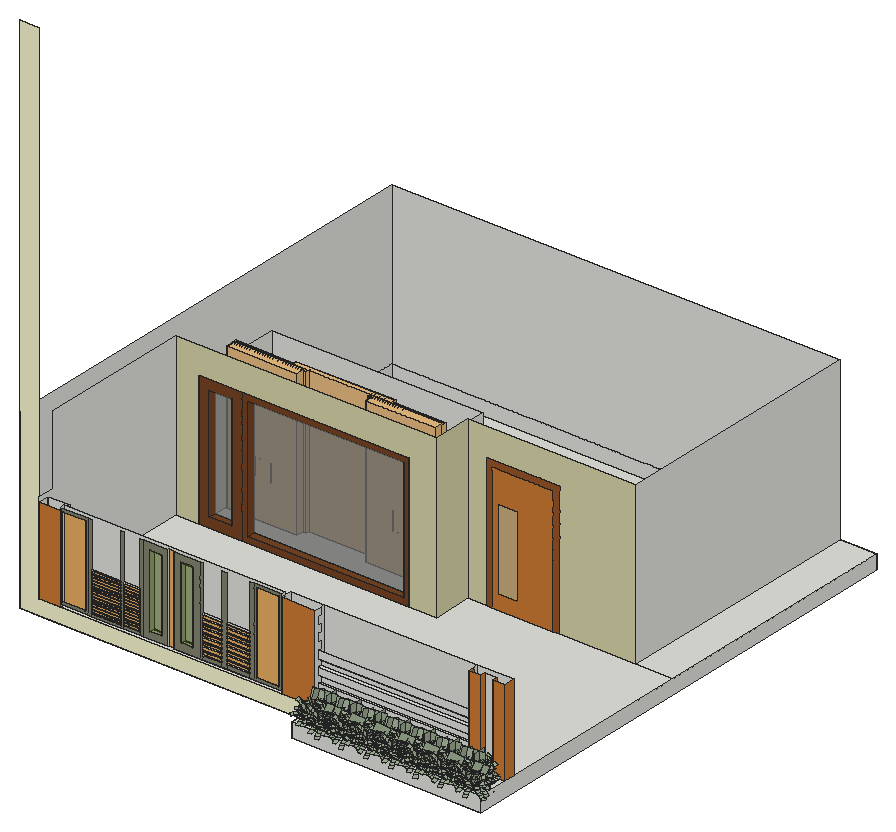
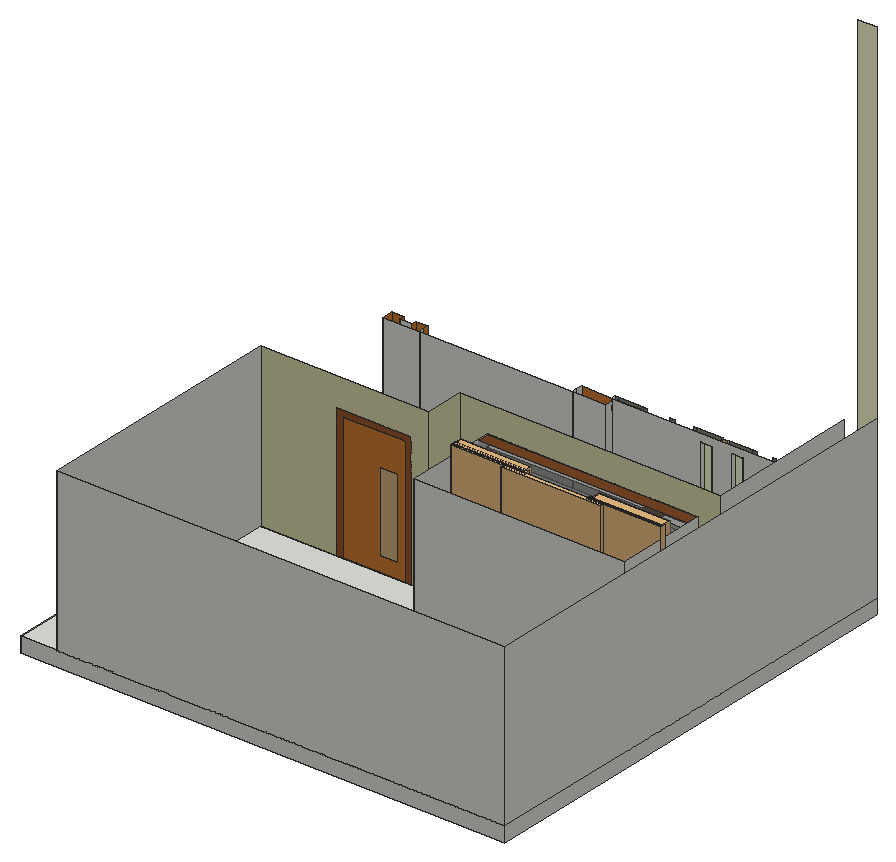
# SketchUp Ruby script. Lengths in inches.
U = 1.inch
M = Sketchup.active_model
def pt(a) = Geom::Point3d.new(a.map { |v| v * U })
def face(e, loops, mat)
  f = e.add_face(loops[0].map { |a| pt(a) })
  loops[1..].each { |l| e.add_face(l.map { |a| pt(a) }).erase! }
  f.material = f.back_material = mat if mat
  f
end
# faces: each face lists its corners as indices into pts; further lists are holes
def faces(e, pts, list, mat = nil) = list.each { |f| face(e, (f[0].is_a?(Array) ? f : [f]).map { |l| l.map { |i| pts[i] } }, mat) }
# xy, xz, yz: faces in a plane at the given z, y or x. An outline is a flat list of corners, or four numbers for a rectangle; further outlines are holes
def ring(l) = l.size == 4 ? [[l[0], l[1]], [l[2], l[1]], [l[2], l[3]], [l[0], l[3]]] : l.each_slice(2).to_a
def flat(e, list, mat, &to3) = list.each { |f| face(e, (f[0].is_a?(Array) ? f : [f]).map { |l| ring(l).map { |u, v| to3.(u, v) } }, mat) }
def xy(e, z, list, mat = nil) = flat(e, list, mat) { |x, y| [x, y, z] }
def xz(e, y, list, mat = nil) = flat(e, list, mat) { |x, z| [x, y, z] }
def yz(e, x, list, mat = nil) = flat(e, list, mat) { |y, z| [x, y, z] }
def lines(e, pts, list) = list.each { |a, b| e.add_line(pt(pts[a]), pt(pts[b])) }
# prism: a flat outline (further loops are holes) pulled along v
def prism(e, loops, v, mat = nil)
  f = face(e, loops, mat); d = Geom::Vector3d.new(v.map { |x| x * U })
  f.pushpull(f.normal.samedirection?(d) ? d.length : -d.length)
end
def box(e, o, s, mat = nil) = prism(e, [[o, [o[0] + s[0], o[1], o[2]], [o[0] + s[0], o[1] + s[1], o[2]], [o[0], o[1] + s[1], o[2]]]], [0, 0, s[2]], mat)
def at(x, y, z, deg = 0) = Geom::Transformation.translation(pt([x, y, z])) * Geom::Transformation.rotation(ORIGIN, Z_AXIS, deg.degrees)
def axes(o, x, y, z) = Geom::Transformation.new([*x, 0, *y, 0, *z, 0, *pt(o).to_a, 1])
def part(name) = M.definitions.add(name)
# library, detail: a bought-in or finely detailed component or shape, given as its bounding box
def library(name, o, s) = part(name).tap { |d| box(d.entities, o, s) }
def detail(e, o, s) = box(e.add_group.entities, o, s)
def put(e, d, t, mat = nil) = e.add_instance(d, t).tap { |i| i.material = mat if mat }
def group(e, t, mat = nil) = e.add_group.tap { |g| g.transformation = t; g.material = mat if mat }.entities
root = M.entities
M.materials.add("Generic").color = [133, 133, 113]
M.materials.add("Generic\#1").color = [235, 176, 99]
M.materials.add("Generic\#4").color = [217, 213, 170]
M.materials.add("Generic\#7").color = [249, 247, 208]
M.materials.add("[Translucent Glass Dark Green]").color = [62, 91, 5]
M.materials["[Translucent Glass Dark Green]"].alpha = 0.5
M.materials.add("[Translucent Glass Gray]").color = [128, 128, 128]
M.materials["[Translucent Glass Gray]"].alpha = 0.5
M.materials.add("[Wood Bamboo]").color = [206, 124, 53]
M.materials.add("[Wood Cherry Original]").color = [152, 86, 42]
M.materials.add("[Wood Floor Light]").color = [204, 176, 127]
M.materials.add("[Wood Veneer 01]").color = [119, 69, 36]
M.materials.add("hymenocallis littoralis").color = [156, 172, 146]
c1 = part("Group\#856")
xy(c1.entities,7.38,[[0,0,5.5,15.91]],"hymenocallis littoralis")
p = [[5.5,28.78,0],[5.5,26.79,3.44],[0,26.79,3.44],[0,28.78,0],[0,23.75,6],[5.5,23.75,6],
  [0,15.91,7.38],[5.5,15.91,7.38]]
faces(c1.entities,p,[[0,1,2,3],[4,2,1,5],[6,4,5,7]],"hymenocallis littoralis")
c2 = part("Group\#854")
xy(c2.entities,7.38,[[0,0,5.5,15.91],[0,15.91,5.5,23.87]],"hymenocallis littoralis")
p = [[5.5,31.07,4.3],[5.5,27.74,6.47],[0,27.74,6.47],[0,31.07,4.3],[0,23.87,7.38],[5.5,23.87,7.38]]
faces(c2.entities,p,[[0,1,2,3],[4,2,1,5]],"hymenocallis littoralis")
c3 = part("Group\#857")
xy(c3.entities,7.38,[[0,0,5.6,15.91]],"hymenocallis littoralis")
p = [[5.6,28.78,0],[5.6,26.79,3.44],[0,26.79,3.44],[0,28.78,0],[0,23.75,6],[5.6,23.75,6],
  [0,15.91,7.38],[5.6,15.91,7.38]]
faces(c3.entities,p,[[0,1,2,3],[4,2,1,5],[6,4,5,7]],"hymenocallis littoralis")
c4 = part("Group\#855")
put(c4.entities,c2,axes([6.09,8.57,-0.52],[0.446,0.85617,0.26089],[-0.18444,-0.19731,0.96283],[0.87582,-0.47754,0.0699]))
put(c4.entities,c2,axes([6.29,7.28,-1.71],[0.37058,0.92707,-0.05667],[-0.32382,0.19004,0.99128],[0.87712,-0.32925,0.34964]))
put(c4.entities,c2,axes([11.04,16.14,-0.7],[1,0,0],[0,0.16628,1.02662],[0,-1.18456,0.19186]))
c5 = part("Group\#860")
put(c5.entities,c1,axes([24.57,32.05,-1.76],[0.9552,-0.22102,-0.19681],[0.4036,0.95545,0.88585],[-0.00568,-0.67859,0.7345]))
put(c5.entities,c1,axes([23.95,29.24,-2.4],[0,1,0],[-0.76041,0,0.64945],[0.64945,0,0.76041]))
put(c5.entities,c1,axes([24.22,24.72,-0.48],[-0.70711,0.70711,0],[-0.32757,-0.32757,0.80237],[0.61237,0.61237,0.5]))
put(c5.entities,c2,axes([20.66,37.22,-0.63],[1.12361,0.03262,0.39091],[-0.43499,0.29739,0.78777],[0.09852,-1.27434,0.37535]))
put(c5.entities,c1,axes([28.75,24.45,-2.4],[-1,0,0],[0,-0.76041,0.64945],[0,0.64945,0.76041]))
put(c5.entities,c3,axes([30.4,30.98,-3.7],[0.65676,-0.72002,0.22414],[0.55667,0.66341,0.5],[-0.50871,-0.20361,0.83652]))
put(c5.entities,c3,axes([32.41,29.61,-3.7],[0.04029,-0.97372,0.22414],[0.85287,0.15038,0.5],[-0.52057,0.17102,0.83652]))
put(c5.entities,c1,axes([31.89,25.85,-1.76],[-0.92056,0.33739,-0.19681],[-0.5186,-0.89824,0.88585],[0.08952,0.67268,0.7345]))
put(c5.entities,c1,axes([25.55,34.78,-0.48],[0.86603,0.5,0],[-0.25,0.43301,0.86603],[0.43301,-0.75,0.5]))
put(c5.entities,c3,axes([20.4,16.9375,-8.07],[-0.70711,0.70711,0],[-0.35754,-0.35754,0.65422],[1.3987,1.3987,1.52882]))
put(c5.entities,c1,axes([32.86,34.14,-0.48],[0.76604,-0.64279,0],[0.32139,0.38302,0.86603],[-0.55667,-0.66341,0.5]))
put(c5.entities,c1,axes([27.15,34.7,-0.1],[0.82472,-0.17528,-0.53769],[0.53769,0.53769,0.64945],[0.17528,-0.82472,0.53769]))
put(c5.entities,c1,axes([33.58,28.77,-2.4],[0,-1,0],[0.76041,0,0.64945],[-0.64945,0,0.76041]))
put(c5.entities,c1,axes([26.43,23.87,-2.81],[-0.75126,0.04415,0.65853],[0.53769,-0.53769,0.64945],[0.38276,0.84199,0.3802]))
put(c5.entities,c1,axes([28.78,23.98,-2.4],[-1,0,0],[0,-0.76041,0.64945],[0,0.64945,0.76041]))
put(c5.entities,c1,axes([25.39,25.38,-2.4],[-0.70711,0.70711,0],[-0.53769,-0.53769,0.64945],[0.45923,0.45923,0.76041]))
put(c5.entities,c1,axes([27.32,21.63,-0.1],[-0.45923,0.70711,-0.53769],[-0.76041,0,0.64945],[0.45923,0.70711,0.53769]))
put(c5.entities,c1,axes([25.17,27.625,-1.76],[0.56416,0.80187,-0.19681],[-0.66673,0.66673,0.80532],[0.62659,-0.26057,0.7345]))
put(c5.entities,c3,axes([27.59,27.04,-3.96],[-0.8993,-0.06127,0.43301],[0.2962,-0.8138,0.5],[0.32175,0.57791,0.75]))
put(c5.entities,c3,axes([26.98,24.5,-3.18],[-0.5,0.86603,0],[-0.75,-0.43301,0.5],[0.43301,0.25,0.86603]))
put(c5.entities,c3,axes([24.55,27.74,-3.7],[0.29517,0.92878,0.22414],[-0.85287,0.15038,0.5],[0.43068,-0.33875,0.83652]))
put(c5.entities,c3,axes([24.26,29.8,-3.18],[0.76604,0.64279,0],[-0.47317,0.5639,0.425],[0.32139,-0.38302,0.86603]))
put(c5.entities,c3,axes([25.98,32.46,-3.18],[1,0,0],[0,0.86603,0.5],[0,-0.5,0.86603]))
put(c5.entities,c1,axes([28.78,33.57,-2.4],[1,0,0],[0,0.76041,0.64945],[0,-0.64945,0.76041]))
put(c5.entities,c4,at(14.99,21.38,2.5))
put(c5.entities,c2,axes([34.63,26.34,-1.46],[-0.70089,-0.70877,0.07994],[0.4756,-0.38088,0.79293],[-0.53156,0.59378,0.60405]))
put(c5.entities,c2,axes([28.14,16.92,1.8125],[-1.19719,0.6912,0],[-0.09607,-0.16641,0.94244],[0.68444,1.18549,0.17613]))
put(c5.entities,c2,axes([31.5625,35.84,0.97],[0.66765,-1.1564,0.35779],[0.04445,0.30732,0.91033],[-1.20828,-0.64496,0.17012]))
put(c5.entities,c2,axes([38.94,22.51,0.89],[-0.97932,-0.67164,-0.05202],[0.27787,-0.41401,0.90999],[-0.85985,0.93577,0.32097]))
put(c5.entities,c2,axes([38.44,21.09,1.98],[-1.02864,-0.54856,0.2395],[0.33481,0.06999,0.88388],[-0.77261,1.08328,0.06417]))
put(c5.entities,c3,axes([35.02,30.51,-1.3],[-0.17365,-0.98481,0],[0.60224,-0.10619,0.79122],[-0.7792,0.13739,0.61153]))
put(c5.entities,c3,axes([29.41,22.33,-1.3],[-0.93969,0.34202,0],[-0.20915,-0.57465,0.79122],[0.27061,0.74351,0.61153]))
put(c5.entities,c2,axes([19.64,36,-1.62],[1.18194,0.09546,0.08234],[-0.14377,0.68823,0.76313],[0.21457,-1.1326,0.62386]))
put(c5.entities,c3,axes([24.25,24.14,-1.3],[-0.34202,0.93969,0],[-0.57465,-0.20915,0.79122],[0.74351,0.27061,0.61153]))
put(c5.entities,c3,axes([25.98,34.61,-1.3],[1,0,0],[0,0.61153,0.79122],[0,-0.79122,0.61153]))
put(c5.entities,c3,axes([31.16,34.41,-1.64],[0.56518,-0.80224,-0.19234],[0.73413,0.34233,0.72935],[-0.47639,-0.50772,0.71782]))
put(c5.entities,c3,axes([40.52,26.84,-5.82],[-0.42262,-0.90631,0],[0.48019,-0.22391,0.68552],[-1.43418,0.66877,1.22305]))
put(c5.entities,c1,axes([29.86,38.42,-1.01],[0.89064,-0.37013,0.26413],[-0.03924,0.63286,1.01918],[-0.45353,-0.76487,0.45748]))
put(c5.entities,c1,axes([29.34,22.4,-0.48],[-0.99619,-0.08716,0],[0.04358,-0.4981,0.86603],[-0.07548,0.86273,0.5]))
c6 = part("Group\#858")
xz(c6.entities,10.07,[[9.07,0,10.07,31.01],[0,31.01,0,45.12,20.13,45.12,20.13,31.01,10.07,31.01,10.07,32.58,9.07,32.58,9.07,31.01]],"hymenocallis littoralis")
yz(c6.entities,10.07,[[0,31.01,20.13,45.12]],"hymenocallis littoralis")
p = [[9.57,9.2,0],[10.07,10.07,0],[10.07,10.07,31.01],[10.07,10.07,32.58],[9.57,9.2,32.58]]
faces(c6.entities,p,[[0,1,2,3,4]],"hymenocallis littoralis")
c7 = part("cây lá nắng")
put(c7.entities,c5,axes([49.26,-2.75,0],[0.63109,0.63109,0],[-0.63109,0.63109,0],[0,0,0.935]))
g1 = group(c7.entities,at(26.6,-8.68,0))
put(g1,c1,axes([-4.72,35.73,-1.65],[0.74231,0.46334,-0.18402],[-0.34827,0.85768,0.82827],[0.42467,-0.43184,0.68675]))
put(g1,c1,axes([-3.34,33.57,-2.24],[-0.63109,0.63109,0],[-0.47989,-0.47989,0.60723],[0.40986,0.40986,0.71098]))
put(g1,c1,axes([-0.3125,30.89,-0.45],[-0.8925,0,0],[0,-0.41345,0.75022],[0,0.77293,0.4675]))
put(g1,c2,axes([-10.79,39.66,-0.59],[0.68852,0.72969,0.3655],[-0.4622,-0.08684,0.73657],[0.86641,-0.74205,0.35095]))
put(g1,c1,axes([2.71,33.57,-2.24],[-0.63109,-0.63109,0],[0.47989,-0.47989,0.60723],[-0.40986,0.40986,0.71098]))
put(g1,c3,axes([-0.37,38.74,-3.46],[0.86887,-0.03992,0.20957],[-0.06737,0.76999,0.4675],[-0.19255,-0.44954,0.78214]))
put(g1,c3,axes([1.76,39.14,-3.46],[0.63993,-0.58908,0.20957],[0.44333,0.63315,0.4675],[-0.43646,-0.2206,0.78214]))
put(g1,c1,axes([3.81,36.4375,-1.65],[-0.79389,-0.36803,-0.18402],[0.23959,-0.89415,0.82827],[-0.36803,0.48102,0.68675]))
put(g1,c1,axes([-5.83,38.07,-0.45],[0.231,0.86209,0],[-0.43104,0.1155,0.80973],[0.74659,-0.20005,0.4675]))
put(g1,c3,axes([2.18,23.5625,-7.55],[-0.8925,0,0],[0,-0.45128,0.6117],[0,1.76542,1.42944]))
put(g1,c1,axes([-0.8125,42.28,-0.45],[0.8891,0.07779,0],[-0.03889,0.44455,0.80973],[0.06737,-0.76999,0.4675]))
put(g1,c1,axes([-4.76,39.03,-0.09],[0.63109,0.40986,-0.50274],[0,0.67866,0.60723],[0.63109,-0.40986,0.50274]))
put(g1,c1,axes([3.03,39.35,-2.24],[0.63109,-0.63109,0],[0.47989,0.47989,0.60723],[-0.40986,-0.40986,0.71098]))
put(g1,c1,axes([1.61,31.74,-2.625],[-0.50198,-0.44625,0.61573],[0.67866,0,0.60723],[-0.28982,0.77293,0.35549]))
put(g1,c1,axes([3.03,33.3,-2.24],[-0.63109,-0.63109,0],[0.47989,-0.47989,0.60723],[-0.40986,0.40986,0.71098]))
put(g1,c1,axes([0.01,32.04,-2.24],[-0.8925,0,0],[0,-0.67866,0.60723],[0,0.57963,0.71098]))
put(g1,c1,axes([3.59,30.89,-0.09],[-0.73607,0.15643,-0.50274],[-0.47989,-0.47989,0.60723],[-0.15643,0.73607,0.50274]))
put(g1,c1,axes([-1.55,33.32,-1.65],[-0.15002,0.86209,-0.18402],[-0.84154,0,0.75297],[0.55988,0.231,0.68675]))
put(g1,c3,axes([0.35,34.48,-3.71],[-0.52887,-0.60621,0.40487],[0.70051,-0.32665,0.4675],[-0.16166,0.56777,0.70125]))
put(g1,c3,axes([2.61,39.13,-1.74],[-0.86209,0.231,0],[-0.23031,-0.85954,0.15531],[0.03162,0.11799,0.91645]))
put(g1,c3,axes([-2.02,33,-3.46],[-0.39986,0.77243,0.20957],[-0.63315,-0.44333,0.4675],[0.48558,0.05802,0.78214]))
put(g1,c3,axes([-3.49,34.12,-2.97],[0.07779,0.8891,0],[-0.65449,0.05726,0.39737],[0.44455,-0.03889,0.80973]))
put(g1,c3,axes([-4.09,36.88,-2.97],[0.63109,0.63109,0],[-0.54654,0.54654,0.4675],[0.31555,-0.31555,0.80973]))
put(g1,c1,axes([-3.02,39.35,-2.24],[0.63109,0.63109,0],[-0.47989,0.47989,0.60723],[0.40986,-0.40986,0.71098]))
put(g1,c4,axes([-4.03,22.95,2.33],[0.63109,0.63109,0],[-0.63109,0.63109,0],[0,0,0.935]))
put(g1,c2,axes([5.24,38.48,-1.37],[0.00497,-0.88963,0.07474],[0.54052,0.05978,0.74139],[-0.71019,0.03927,0.56479]))
put(g1,c2,axes([7.08,28.4375,1.7],[-1.19175,-0.31933,0],[0.04439,-0.16565,0.88118],[-0.31621,1.1801,0.16468]))
put(g1,c2,axes([-2.7,42.54,0.91],[1.15114,-0.30845,0.33454],[-0.1659,0.22199,0.85115],[-0.3555,-1.16957,0.15907]))
put(g1,c2,axes([10.37,38.78,0.83],[-0.19417,-1.04191,-0.04864],[0.43664,-0.08592,0.85084],[-1.1332,0.04791,0.30011]))
put(g1,c2,axes([10.95,37.5625,1.85],[-0.30298,-0.99536,0.22393],[0.16713,0.25547,0.82643],[-1.17124,0.19607,0.06]))
put(g1,c3,axes([2.84,41.36,-1.22],[0.51192,-0.73109,0],[0.44708,0.31305,0.73979],[-0.57846,-0.40504,0.57178]))
put(g1,c3,axes([4.47,32.65,-1.22],[-0.80888,-0.37719,0],[0.23066,-0.49465,0.73979],[-0.29844,0.64,0.57178]))
put(g1,c2,axes([-10.32,35.12,-1.51],[0.68567,0.80616,0.07699],[-0.52507,0.3436,0.71352],[0.85019,-0.57936,0.58331]))
put(g1,c3,axes([0.07,30.54,-1.22],[-0.80888,0.37719,0],[-0.23066,-0.49465,0.73979],[0.29844,0.64,0.57178]))
put(g1,c3,axes([-5.45,38.24,-1.22],[0.63109,0.63109,0],[-0.38593,0.38593,0.73979],[0.49934,-0.49934,0.57178]))
put(g1,c3,axes([-2.05,41.38,-1.53],[0.86296,-0.14961,-0.17984],[0.24726,0.67935,0.68194],[0.01977,-0.62107,0.67116]))
put(g1,c3,axes([8.63,42.51,-5.4375],[0.30525,-0.83868,0],[0.44435,0.16173,0.64096],[-1.32716,-0.48305,1.14356]))
put(g1,c1,axes([-5.4,43.09,-0.94],[0.79566,0.32849,0.24696],[-0.42416,0.37462,0.95293],[0.19648,-0.76892,0.42774]))
put(g1,c1,axes([4.38,32.65,-0.45],[-0.57369,-0.68369,0],[0.34185,-0.28684,0.80973],[-0.5921,0.49683,0.4675]))
put(g1,c3,axes([-2,33.84,-0.15],[-0.24601,0.85793,0],[-0.85539,-0.24528,0.15531],[0.11742,0.03367,0.91645]))
put(g1,c3,axes([0.17,30.83,-4.47],[-0.24601,0.85793,0],[-0.85539,-0.24528,0.15531],[0.11742,0.03367,0.91645]))
put(g1,c3,axes([-1.97,32.18,-4.47],[0.58524,0.67383,0],[-0.67184,0.58351,0.15531],[0.09222,-0.0801,0.91645]))
put(g1,c3,axes([-2,34.71,-4.47],[0.88392,-0.12346,0],[0.12309,0.88131,0.15531],[-0.0169,-0.12098,0.91645]))
put(g1,c3,axes([0.11,36.12,-4.47],[0.37822,-0.8084,0],[0.80601,0.37711,0.15531],[-0.11064,-0.05177,0.91645]))
put(c7.entities,c6,axes([29.71,14.29,6.94],[0.425,0.73612,0],[-0.6771,0.39092,-0.33349],[-0.26859,0.15507,0.72712]))
put(c7.entities,c6,axes([42.0625,26.12,6.94],[0.85,0,0],[0,0.78185,-0.33349],[0,0.33349,0.78185]))
put(c7.entities,c5,axes([7.3125,23.0625,0],[0.8925,0,0],[0,0.8925,0],[0,0,0.935]))
put(c7.entities,c6,axes([24.4375,40.23,2.05],[0.85,0,0],[0,0.85,0],[0,0,0.85]))
c8 = part("Planting+101")
put(c8.entities,c7,axes([21.34,32.96,-4.59],[0,-0.71,0],[-0.71,0,0],[0,0,0.71]))
c9 = library("Group14",[-64.97,9.24,0.31],[138.52,9.93,292.57])
c10 = library("Group16",[86.37,-10.76,76.46],[21.79,14.87,35.97])
c11 = library("Group22",[48.82,-10.91,0.23],[97.72,18.57,293.12])
c12 = library("Group24",[44.03,2.01,0.26],[103.73,11,292.35])
c13 = library("Group27",[-106.21,-10.76,76.46],[21.8,14.87,35.97])
c14 = library("Group35",[-145.81,2.01,0.26],[103.73,11,292.35])
c15 = library("Group33",[-144.59,-10.91,0.23],[97.72,18.57,293.12])
c16 = part("rem (1)")
g2 = group(c16.entities,at(-145.81,-10.91,0.23))
put(g2,c9,at(145.81,10.91,-0.23))
put(g2,c10,at(145.81,10.91,-0.23))
put(g2,c11,at(145.81,10.91,-0.23))
put(g2,c12,at(145.81,10.91,-0.23))
put(g2,c13,at(145.81,10.91,-0.23))
put(g2,c14,at(145.81,10.91,-0.23))
put(g2,c15,at(145.81,10.91,-0.23))
c17 = part("Group\#5")
xz(c17.entities,0,[[0,0,11.45,75.29]],"[Translucent Glass Dark Green]")
xy(root,-37.25,[[304.6875,37.125,304.6875,67.875,19.1875,67.875,19.1875,244.125,500.125,244.125,500.125,37.125],[0,67.875,0,547.875,500.125,547.875,500.125,244.125,19.1875,244.125,19.1875,67.875]])
xy(root,-29.125,[[309.97,40.97,494.84,64.03]])
xy(root,-21.875,[[[304.6875,37.125,500.125,37.125,500.125,67.875,487.6875,67.875,487.6875,73.0625,475.25,73.0625,475.25,67.875,462.8125,67.875,462.8125,71.375,304.6875,71.375],[309.97,40.97,494.84,64.03]],[19.1875,67.875,41.625,79.3125],[41.625,67.875,269.875,79.3125],[269.875,67.875,304.6875,79.3125],[462.8125,67.875,475.25,67.875,475.25,73.0625,487.6875,73.0625,487.6875,67.875,500.125,67.875,500.125,79.3125,462.8125,79.3125],
  [304.6875,71.375,462.8125,73.0625],[304.6875,73.0625,462.8125,79.3125],[19.1875,79.3125,500.125,79.3125,500.125,284.5625,288.89,284.5625,288.89,244.125,19.1875,244.125],[43.125,244.125,260.5625,338.6875],[462.8125,284.5625,500.125,547.875]])
xy(root,-18.875,[[41.625,67.875,41.625,72.625,269.875,72.625,269.875,67.875,158.75,67.875,158.75,68.625,152.75,68.625,152.75,67.875]])
xy(root,-16.375,[[304.6875,71.375,462.8125,74.375]])
xy(root,-16.14,[[44.36,67.875,67.42,68.625]])
xy(root,-16.125,[[74.16,67.875,103.6875,68.625],[107.25,67.875,123.28,68.625]])
xy(root,-16.11,[[244.11,67.875,267.11,68.625]])
xy(root,-15.3125,[[188.84,67.875,208,68.625],[212.8125,67.875,236.91,68.625]],"Generic")
xy(root,-14.875,[[74.16,67.875,103.6875,68.625],[107.25,67.875,123.28,68.625]])
xy(root,-13.5,[[188.84,67.875,208,68.625],[212.8125,67.875,236.91,68.625]],"Generic")
xy(root,-13.125,[[74.16,67.875,103.6875,68.625],[107.25,67.875,123.28,68.625]])
xy(root,-11.875,[[74.16,67.875,103.6875,68.625],[107.25,67.875,123.28,68.625]])
xy(root,-11.83,[[134.26,67.875,145.71,72.625]])
xy(root,-11.3125,[[166.3125,67.875,177.72,72.625]])
xy(root,-11.125,[[188.84,67.875,208,68.625],[212.8125,67.875,236.91,68.625]],"Generic")
xy(root,-10.125,[[74.16,67.875,103.6875,68.625],[107.25,67.875,123.28,68.625]])
xy(root,-9.3125,[[188.84,67.875,208,68.625],[212.8125,67.875,236.91,68.625]],"Generic")
xy(root,-8.9375,[[304.6875,71.375,462.8125,74.375]])
xy(root,-8.875,[[74.16,67.875,103.6875,68.625],[107.25,67.875,123.28,68.625]])
xy(root,-7.125,[[74.16,67.875,103.6875,68.625],[107.25,67.875,123.28,68.625]])
xy(root,-6.9375,[[188.84,67.875,208,68.625],[212.8125,67.875,236.91,68.625]],"Generic")
xy(root,-5.875,[[74.16,67.875,103.6875,68.625],[107.25,67.875,123.28,68.625]])
xy(root,-5.125,[[188.84,67.875,208,68.625],[212.8125,67.875,236.91,68.625]],"Generic")
xy(root,-4.125,[[74.16,67.875,103.6875,68.625],[107.25,67.875,123.28,68.625]])
xy(root,-2.875,[[74.16,67.875,103.6875,68.625],[107.25,67.875,123.28,68.625]])
xy(root,-2.75,[[188.84,67.875,208,68.625],[212.8125,67.875,236.91,68.625]],"Generic")
xy(root,-1.125,[[74.16,67.875,103.6875,68.625],[107.25,67.875,123.28,68.625]])
xy(root,-1.0625,[[304.6875,71.375,462.8125,74.375]])
xy(root,-0.9375,[[188.84,67.875,208,68.625],[212.8125,67.875,236.91,68.625]],"Generic")
xy(root,0.125,[[74.16,67.875,103.6875,68.625],[107.25,67.875,123.28,68.625]])
xy(root,1.4375,[[188.84,67.875,208,68.625],[212.8125,67.875,236.91,68.625]],"Generic")
xy(root,1.875,[[74.16,67.875,103.6875,68.625],[107.25,67.875,123.28,68.625]])
xy(root,3.125,[[74.16,67.875,103.6875,68.625],[107.25,67.875,123.28,68.625]])
xy(root,3.25,[[188.84,67.875,208,68.625],[212.8125,67.875,236.91,68.625]],"Generic")
xy(root,4.875,[[74.16,67.875,103.6875,68.625],[107.25,67.875,123.28,68.625]])
xy(root,5.625,[[188.84,67.875,208,68.625],[212.8125,67.875,236.91,68.625]],"Generic")
xy(root,6.125,[[74.16,67.875,103.6875,68.625],[107.25,67.875,123.28,68.625]])
xy(root,6.375,[[304.6875,71.375,462.8125,74.375]])
xy(root,7.4375,[[188.84,67.875,208,68.625],[212.8125,67.875,236.91,68.625]],"Generic")
xy(root,7.875,[[74.16,67.875,103.6875,68.625],[107.25,67.875,123.28,68.625]])
xy(root,9.125,[[74.16,67.875,103.6875,68.625],[107.25,67.875,123.28,68.625]])
xy(root,9.8125,[[188.84,67.875,208,68.625],[212.8125,67.875,236.91,68.625]],"Generic")
xy(root,10.875,[[74.16,67.875,103.6875,68.625],[107.25,67.875,123.28,68.625]])
xy(root,11.625,[[188.84,67.875,208,68.625],[212.8125,67.875,236.91,68.625]],"Generic")
xy(root,12.125,[[74.16,67.875,103.6875,68.625],[107.25,67.875,123.28,68.625]])
xy(root,13.875,[[74.16,67.875,103.6875,68.625],[107.25,67.875,123.28,68.625]])
xy(root,14,[[188.84,67.875,208,68.625],[212.8125,67.875,236.91,68.625]],"Generic")
xy(root,14.25,[[304.6875,71.375,462.8125,74.375]])
xy(root,15.125,[[74.16,67.875,103.6875,68.625],[107.25,67.875,123.28,68.625]])
xy(root,15.8125,[[188.84,67.875,208,68.625],[212.8125,67.875,236.91,68.625]],"Generic")
xy(root,16.875,[[74.16,67.875,103.6875,68.625],[107.25,67.875,123.28,68.625]])
xy(root,18.125,[[74.16,67.875,103.6875,68.625],[107.25,67.875,123.28,68.625]])
xy(root,18.1875,[[188.84,67.875,208,68.625],[212.8125,67.875,236.91,68.625]],"Generic")
xy(root,19.875,[[74.16,67.875,103.6875,68.625],[107.25,67.875,123.28,68.625]])
xy(root,20,[[188.84,67.875,208,68.625],[212.8125,67.875,236.91,68.625]],"Generic")
xy(root,21.125,[[74.16,67.875,103.6875,68.625],[107.25,67.875,123.28,68.625]])
xy(root,21.6875,[[304.6875,71.375,462.8125,74.375]])
xy(root,22.375,[[188.84,67.875,208,68.625],[212.8125,67.875,236.91,68.625]],"Generic")
xy(root,22.875,[[74.16,67.875,103.6875,68.625],[107.25,67.875,123.28,68.625]])
xz(root,37.125,[[304.6875,-37.25,500.125,-21.875]])
xz(root,40.97,[[309.97,-29.125,494.84,-21.875]])
xz(root,64.03,[[309.97,-29.125,494.84,-21.875]])
xz(root,67.875,[[[41.625,-18.875,70.16,70.5],[44.36,-16.14,67.42,67.76]],[70.16,-18.875,74.16,70.5],[74.16,-18.875,103.6875,-16.125],[103.6875,-18.875,107.25,70.5],[107.25,-18.875,123.28,-16.125],
  [123.28,-18.875,127.22,70.5],[[127.22,-18.875,152.75,70.5],[134.26,-11.83,145.71,63.46]],[[158.75,-18.875,185.28,70.5],[166.3125,-11.3125,177.72,62.9375]],[185.28,-18.875,188.84,70.5],[188.84,-18.875,208,-15.3125],
  [208,-18.875,212.8125,70.5],[212.8125,-18.875,236.91,-15.3125],[236.91,-18.875,241.34,70.5],[[241.34,-18.875,269.875,70.5],[244.11,-16.11,267.11,67.73]]],"Generic")
xz(root,67.875,[[74.16,-14.875,103.6875,-13.125],[107.25,-14.875,123.28,-13.125],[188.84,-13.5,208,-11.125],[212.8125,-13.5,236.91,-11.125],[74.16,-11.875,103.6875,-10.125],
  [107.25,-11.875,123.28,-10.125],[188.84,-9.3125,208,-6.9375],[212.8125,-9.3125,236.91,-6.9375],[74.16,-8.875,103.6875,-7.125],[107.25,-8.875,123.28,-7.125],
  [74.16,-5.875,103.6875,-4.125],[107.25,-5.875,123.28,-4.125],[188.84,-5.125,208,-2.75],[212.8125,-5.125,236.91,-2.75],[74.16,-2.875,103.6875,-1.125],
  [107.25,-2.875,123.28,-1.125],[188.84,-0.9375,208,1.4375],[212.8125,-0.9375,236.91,1.4375],[74.16,0.125,103.6875,1.875],[107.25,0.125,123.28,1.875],
  [74.16,3.125,103.6875,4.875],[107.25,3.125,123.28,4.875],[188.84,3.25,208,5.625],[212.8125,3.25,236.91,5.625],[74.16,6.125,103.6875,7.875],
  [107.25,6.125,123.28,7.875],[188.84,7.4375,208,9.8125],[212.8125,7.4375,236.91,9.8125],[74.16,9.125,103.6875,10.875],[107.25,9.125,123.28,10.875],
  [188.84,11.625,208,14],[212.8125,11.625,236.91,14],[74.16,12.125,103.6875,13.875],[107.25,12.125,123.28,13.875],[74.16,15.125,103.6875,16.875],
  [107.25,15.125,123.28,16.875],[188.84,15.8125,208,18.1875],[212.8125,15.8125,236.91,18.1875],[74.16,18.125,103.6875,19.875],[107.25,18.125,123.28,19.875],
  [188.84,20,208,22.375],[212.8125,20,236.91,22.375],[74.16,21.125,103.6875,22.875],[107.25,21.125,123.28,22.875]],"Generic\#1")
xz(root,67.875,[[0,-37.25,304.6875,-37.25,304.6875,-21.875,19.1875,-21.875,19.1875,506.6875,0,506.6875]],"Generic\#7")
xz(root,67.875,[[19.1875,-21.875,41.625,67.5],[269.875,-21.875,304.6875,67.5],[462.8125,-21.875,475.25,67.5],[487.6875,-21.875,500.125,67.5]],"[Wood Bamboo]")
xz(root,68.625,[[74.16,-16.125,103.6875,-14.875],[107.25,-16.125,123.28,-14.875],[188.84,-15.3125,208,-13.5],[212.8125,-15.3125,236.91,-13.5],[74.16,-13.125,103.6875,-11.875],
  [107.25,-13.125,123.28,-11.875],[188.84,-11.125,208,-9.3125],[212.8125,-11.125,236.91,-9.3125],[74.16,-10.125,103.6875,-8.875],[107.25,-10.125,123.28,-8.875],
  [74.16,-7.125,103.6875,-5.875],[107.25,-7.125,123.28,-5.875],[188.84,-6.9375,208,-5.125],[212.8125,-6.9375,236.91,-5.125],[74.16,-4.125,103.6875,-2.875],
  [107.25,-4.125,123.28,-2.875],[188.84,-2.75,208,-0.9375],[212.8125,-2.75,236.91,-0.9375],[74.16,-1.125,103.6875,0.125],[107.25,-1.125,123.28,0.125],
  [188.84,1.4375,208,3.25],[212.8125,1.4375,236.91,3.25],[74.16,1.875,103.6875,3.125],[107.25,1.875,123.28,3.125],[74.16,4.875,103.6875,6.125],
  [107.25,4.875,123.28,6.125],[188.84,5.625,208,7.4375],[212.8125,5.625,236.91,7.4375],[74.16,7.875,103.6875,9.125],[107.25,7.875,123.28,9.125],
  [188.84,9.8125,208,11.625],[212.8125,9.8125,236.91,11.625],[74.16,10.875,103.6875,12.125],[107.25,10.875,123.28,12.125],[74.16,13.875,103.6875,15.125],
  [107.25,13.875,123.28,15.125],[188.84,14,208,15.8125],[212.8125,14,236.91,15.8125],[74.16,16.875,103.6875,18.125],[107.25,16.875,123.28,18.125],
  [188.84,18.1875,208,20],[212.8125,18.1875,236.91,20],[74.16,19.875,103.6875,21.125],[107.25,19.875,123.28,21.125],[188.84,22.375,208,24.1875],
  [212.8125,22.375,236.91,24.1875],[74.16,22.875,103.6875,24.125],[107.25,22.875,123.28,24.125]])
xz(root,68.625,[[152.75,-18.875,158.75,70.5],[44.36,-16.14,67.42,67.76],[244.11,-16.11,267.11,67.73]],"Generic\#1")
xz(root,71.375,[[304.6875,-21.875,462.8125,-16.375],[304.6875,-8.9375,462.8125,-1.0625],[304.6875,6.375,462.8125,14.25],[304.6875,21.6875,462.8125,29.5625]])
xz(root,72.625,[[[41.625,-18.875,269.875,70.5],[134.26,-11.83,145.71,63.46],[166.3125,-11.3125,177.72,62.9375]]])
xz(root,73.0625,[[304.6875,-39.5625,462.8125,-31.6875],[304.6875,-24.25,462.8125,-21.875],[475.25,-21.875,487.6875,67.5]])
xz(root,74.375,[[304.6875,-16.375,462.8125,-8.9375],[304.6875,-1.0625,462.8125,6.375],[304.6875,14.25,462.8125,21.6875]])
xz(root,79.3125,[[19.1875,-21.875,41.625,67.5],[269.875,-21.875,304.6875,67.5],[304.6875,-21.875,462.8125,67.5],[462.8125,-21.875,500.125,67.5]])
xz(root,244.125,[[19.1875,-21.875,43.125,-21.875,43.125,115.9375,260.5625,115.9375,260.5625,-21.875,288.89,-21.875,288.89,144,19.1875,144]],"Generic\#4")
xz(root,284.5625,[[288.89,-21.875,307.17,-21.875,307.17,115.125,383.73,115.125,383.73,-21.875,462.8125,-21.875,462.8125,144,288.89,144]],"Generic\#4")
xz(root,284.5625,[[[313.94,-21.875,376.96,108.36],[321.2,-6.58,339.83,76.04]]],"[Wood Bamboo]")
xz(root,284.5625,[[307.17,-21.875,313.94,-21.875,313.94,108.36,376.96,108.36,376.96,-21.875,383.73,-21.875,383.73,115.125,307.17,115.125]],"[Wood Cherry Original]")
xz(root,284.5625,[[321.2,-6.58,339.83,76.04]],"[Wood Floor Light]")
xz(root,338.6875,[[43.125,-21.875,260.5625,115.9375]])
xz(root,547.875,[[0,-37.25,500.125,-21.875],[0,-21.875,462.8125,144]])
yz(root,0,[[67.875,-37.25,547.875,-21.875],[67.875,-21.875,547.875,144]])
yz(root,19.1875,[[67.875,-21.875,79.3125,67.5],[79.3125,-21.875,244.125,-21.875,244.125,144,85.3125,144,85.3125,72.125,67.875,72.125,67.875,67.5,79.3125,67.5]])
yz(root,41.625,[[67.875,-21.875,79.3125,67.5],[67.875,-18.875,72.625,70.5]])
yz(root,43.125,[[244.125,-21.875,338.6875,115.9375]])
yz(root,44.36,[[67.875,-16.14,68.625,67.76]])
yz(root,67.42,[[67.875,-16.14,68.625,67.76]])
yz(root,74.16,[[67.875,-16.125,68.625,-14.875],[67.875,-13.125,68.625,-11.875],[67.875,-10.125,68.625,-8.875],[67.875,-7.125,68.625,-5.875],[67.875,-4.125,68.625,-2.875],
  [67.875,-1.125,68.625,0.125],[67.875,1.875,68.625,3.125],[67.875,4.875,68.625,6.125],[67.875,7.875,68.625,9.125],[67.875,10.875,68.625,12.125],
  [67.875,13.875,68.625,15.125],[67.875,16.875,68.625,18.125],[67.875,19.875,68.625,21.125],[67.875,22.875,68.625,24.125]])
yz(root,103.6875,[[67.875,-16.125,68.625,-14.875],[67.875,-13.125,68.625,-11.875],[67.875,-10.125,68.625,-8.875],[67.875,-7.125,68.625,-5.875],[67.875,-4.125,68.625,-2.875],
  [67.875,-1.125,68.625,0.125],[67.875,1.875,68.625,3.125],[67.875,4.875,68.625,6.125],[67.875,7.875,68.625,9.125],[67.875,10.875,68.625,12.125],
  [67.875,13.875,68.625,15.125],[67.875,16.875,68.625,18.125],[67.875,19.875,68.625,21.125],[67.875,22.875,68.625,24.125]])
yz(root,107.25,[[67.875,-16.125,68.625,-14.875],[67.875,-13.125,68.625,-11.875],[67.875,-10.125,68.625,-8.875],[67.875,-7.125,68.625,-5.875],[67.875,-4.125,68.625,-2.875],
  [67.875,-1.125,68.625,0.125],[67.875,1.875,68.625,3.125],[67.875,4.875,68.625,6.125],[67.875,7.875,68.625,9.125],[67.875,10.875,68.625,12.125],
  [67.875,13.875,68.625,15.125],[67.875,16.875,68.625,18.125],[67.875,19.875,68.625,21.125],[67.875,22.875,68.625,24.125]])
yz(root,123.28,[[67.875,-16.125,68.625,-14.875],[67.875,-13.125,68.625,-11.875],[67.875,-10.125,68.625,-8.875],[67.875,-7.125,68.625,-5.875],[67.875,-4.125,68.625,-2.875],
  [67.875,-1.125,68.625,0.125],[67.875,1.875,68.625,3.125],[67.875,4.875,68.625,6.125],[67.875,7.875,68.625,9.125],[67.875,10.875,68.625,12.125],
  [67.875,13.875,68.625,15.125],[67.875,16.875,68.625,18.125],[67.875,19.875,68.625,21.125],[67.875,22.875,68.625,24.125]])
yz(root,134.26,[[67.875,-11.83,72.625,63.46]])
yz(root,145.71,[[67.875,-11.83,72.625,63.46]])
yz(root,152.75,[[67.875,-18.875,68.625,70.5]])
yz(root,158.75,[[67.875,-18.875,68.625,70.5]])
yz(root,166.3125,[[67.875,-11.3125,72.625,62.9375]])
yz(root,177.72,[[67.875,-11.3125,72.625,62.9375]])
yz(root,188.84,[[67.875,-15.3125,68.625,-13.5],[67.875,-11.125,68.625,-9.3125],[67.875,-6.9375,68.625,-5.125],[67.875,-2.75,68.625,-0.9375],[67.875,1.4375,68.625,3.25],
  [67.875,5.625,68.625,7.4375],[67.875,9.8125,68.625,11.625],[67.875,14,68.625,15.8125],[67.875,18.1875,68.625,20],[67.875,22.375,68.625,24.1875]])
yz(root,208,[[67.875,-15.3125,68.625,-13.5],[67.875,-11.125,68.625,-9.3125],[67.875,-6.9375,68.625,-5.125],[67.875,-2.75,68.625,-0.9375],[67.875,1.4375,68.625,3.25],
  [67.875,5.625,68.625,7.4375],[67.875,9.8125,68.625,11.625],[67.875,14,68.625,15.8125],[67.875,18.1875,68.625,20],[67.875,22.375,68.625,24.1875]])
yz(root,212.8125,[[67.875,-15.3125,68.625,-13.5],[67.875,-11.125,68.625,-9.3125],[67.875,-6.9375,68.625,-5.125],[67.875,-2.75,68.625,-0.9375],[67.875,1.4375,68.625,3.25],
  [67.875,5.625,68.625,7.4375],[67.875,9.8125,68.625,11.625],[67.875,14,68.625,15.8125],[67.875,18.1875,68.625,20],[67.875,22.375,68.625,24.1875]])
yz(root,236.91,[[67.875,-15.3125,68.625,-13.5],[67.875,-11.125,68.625,-9.3125],[67.875,-6.9375,68.625,-5.125],[67.875,-2.75,68.625,-0.9375],[67.875,1.4375,68.625,3.25],
  [67.875,5.625,68.625,7.4375],[67.875,9.8125,68.625,11.625],[67.875,14,68.625,15.8125],[67.875,18.1875,68.625,20],[67.875,22.375,68.625,24.1875]])
yz(root,244.11,[[67.875,-16.11,68.625,67.73]])
yz(root,260.5625,[[244.125,-21.875,338.6875,115.9375]])
yz(root,267.11,[[67.875,-16.11,68.625,67.73]])
yz(root,269.875,[[67.875,-21.875,79.3125,67.5],[67.875,-18.875,72.625,70.5]])
yz(root,288.89,[[244.125,-21.875,284.5625,144]],"Generic\#4")
yz(root,304.6875,[[37.125,-37.25,67.875,-21.875],[67.875,-21.875,71.375,-21.875,71.375,-16.375,74.375,-16.375,74.375,-8.9375,71.375,-8.9375,71.375,-1.0625,74.375,-1.0625,74.375,6.375,71.375,6.375,71.375,14.25,74.375,14.25,74.375,21.6875,71.375,21.6875,71.375,29.5625,74.375,29.5625,74.375,37,71.375,37,71.375,44.875,74.375,44.875,74.375,52.3125,71.375,52.3125,71.375,60.1875,74.375,60.1875,74.375,67.5,67.875,67.5],[71.375,-21.875,79.3125,-21.875,79.3125,67.5,74.375,67.5,74.375,60.1875,71.375,60.1875,71.375,52.3125,74.375,52.3125,74.375,44.875,71.375,44.875,71.375,37,74.375,37,74.375,29.5625,71.375,29.5625,71.375,21.6875,74.375,21.6875,74.375,14.25,71.375,14.25,71.375,6.375,74.375,6.375,74.375,-1.0625,71.375,-1.0625,71.375,-8.9375,74.375,-8.9375,74.375,-16.375,71.375,-16.375]])
yz(root,309.97,[[40.97,-29.125,64.03,-21.875]])
yz(root,462.8125,[[71.375,-21.875,71.375,-16.375,74.375,-16.375,74.375,-8.9375,71.375,-8.9375,71.375,-1.0625,74.375,-1.0625,74.375,6.375,71.375,6.375,71.375,14.25,74.375,14.25,74.375,21.6875,71.375,21.6875,71.375,29.5625,74.375,29.5625,74.375,37,71.375,37,71.375,44.875,74.375,44.875,74.375,52.3125,71.375,52.3125,71.375,60.1875,74.375,60.1875,74.375,67.5,79.3125,67.5,79.3125,-21.875],[284.5625,-21.875,547.875,144]])
yz(root,462.8125,[[67.875,-21.875,67.875,67.5,74.375,67.5,74.375,60.1875,71.375,60.1875,71.375,52.3125,74.375,52.3125,74.375,44.875,71.375,44.875,71.375,37,74.375,37,74.375,29.5625,71.375,29.5625,71.375,21.6875,74.375,21.6875,74.375,14.25,71.375,14.25,71.375,6.375,74.375,6.375,74.375,-1.0625,71.375,-1.0625,71.375,-8.9375,74.375,-8.9375,74.375,-16.375,71.375,-16.375,71.375,-21.875]],"[Wood Bamboo]")
yz(root,475.25,[[67.875,-21.875,73.0625,67.5]],"[Wood Bamboo]")
yz(root,487.6875,[[67.875,-21.875,73.0625,67.5]],"[Wood Bamboo]")
yz(root,494.84,[[40.97,-29.125,64.03,-21.875]])
yz(root,500.125,[[37.125,-37.25,547.875,-21.875]])
yz(root,500.125,[[67.875,-21.875,79.3125,67.5]],"[Wood Bamboo]")
p = [[19.1875,244.125,-21.875],[19.1875,244.125,-37.25]]
lines(root,p,[[0,1]])
put(root,c8,at(318.74,45.43,-20.23,-90))
put(root,c8,at(344.24,45.43,-20.23,-90))
put(root,c8,at(369.74,45.43,-20.23,-90))
put(root,c8,at(395.24,45.43,-20.23,-90))
put(root,c8,at(420.74,45.43,-20.23,-90))
put(root,c8,at(446.24,45.43,-20.23,-90))
put(root,c8,at(471.74,45.43,-20.23,-90))
g3 = group(root,at(43.125,244.125,-21.875))
xy(g3,0,[[0,0,217.4375,12.75]])
xy(g3,5.87,[[50.43,0,211.57,7.75]],"[Wood Veneer 01]")
xy(g3,10.14,[[10.14,0,34.42,7.75]],"[Wood Veneer 01]")
xy(g3,127.67,[[10.14,0,34.42,7.75]])
xy(g3,131.94,[[50.43,0,211.57,7.75]])
xy(g3,137.8125,[[0,0,217.4375,12.75]],"[Wood Veneer 01]")
xz(g3,0,[[[0,0,44.5625,137.8125],[10.14,10.14,34.42,127.67]],[[44.5625,0,217.4375,137.8125],[50.43,5.87,211.57,131.94]]],"[Wood Veneer 01]")
xz(g3,7.75,[[50.43,5.87,211.57,131.94],[10.14,10.14,34.42,127.67]],"[Translucent Glass Gray]")
xz(g3,12.75,[[0,0,217.4375,137.8125]],"[Translucent Glass Gray]")
yz(g3,0,[[0,0,12.75,137.8125]],"[Wood Veneer 01]")
yz(g3,10.14,[[0,10.14,7.75,127.67]],"[Wood Veneer 01]")
yz(g3,34.42,[[0,10.14,7.75,127.67]],"[Wood Veneer 01]")
yz(g3,50.43,[[0,5.87,7.75,131.94]],"[Wood Veneer 01]")
yz(g3,211.57,[[0,5.87,7.75,131.94]],"[Wood Veneer 01]")
yz(g3,217.4375,[[0,0,12.75,137.8125]],"[Wood Veneer 01]")
put(root,c16,axes([151.12,285.48,-21.99],[0.74066,0,0],[0,0.51,0],[0,0,0.51]))
put(root,c17,at(134.26,67.875,-11.83))
put(root,c17,at(166.27,67.875,-11.3125))
